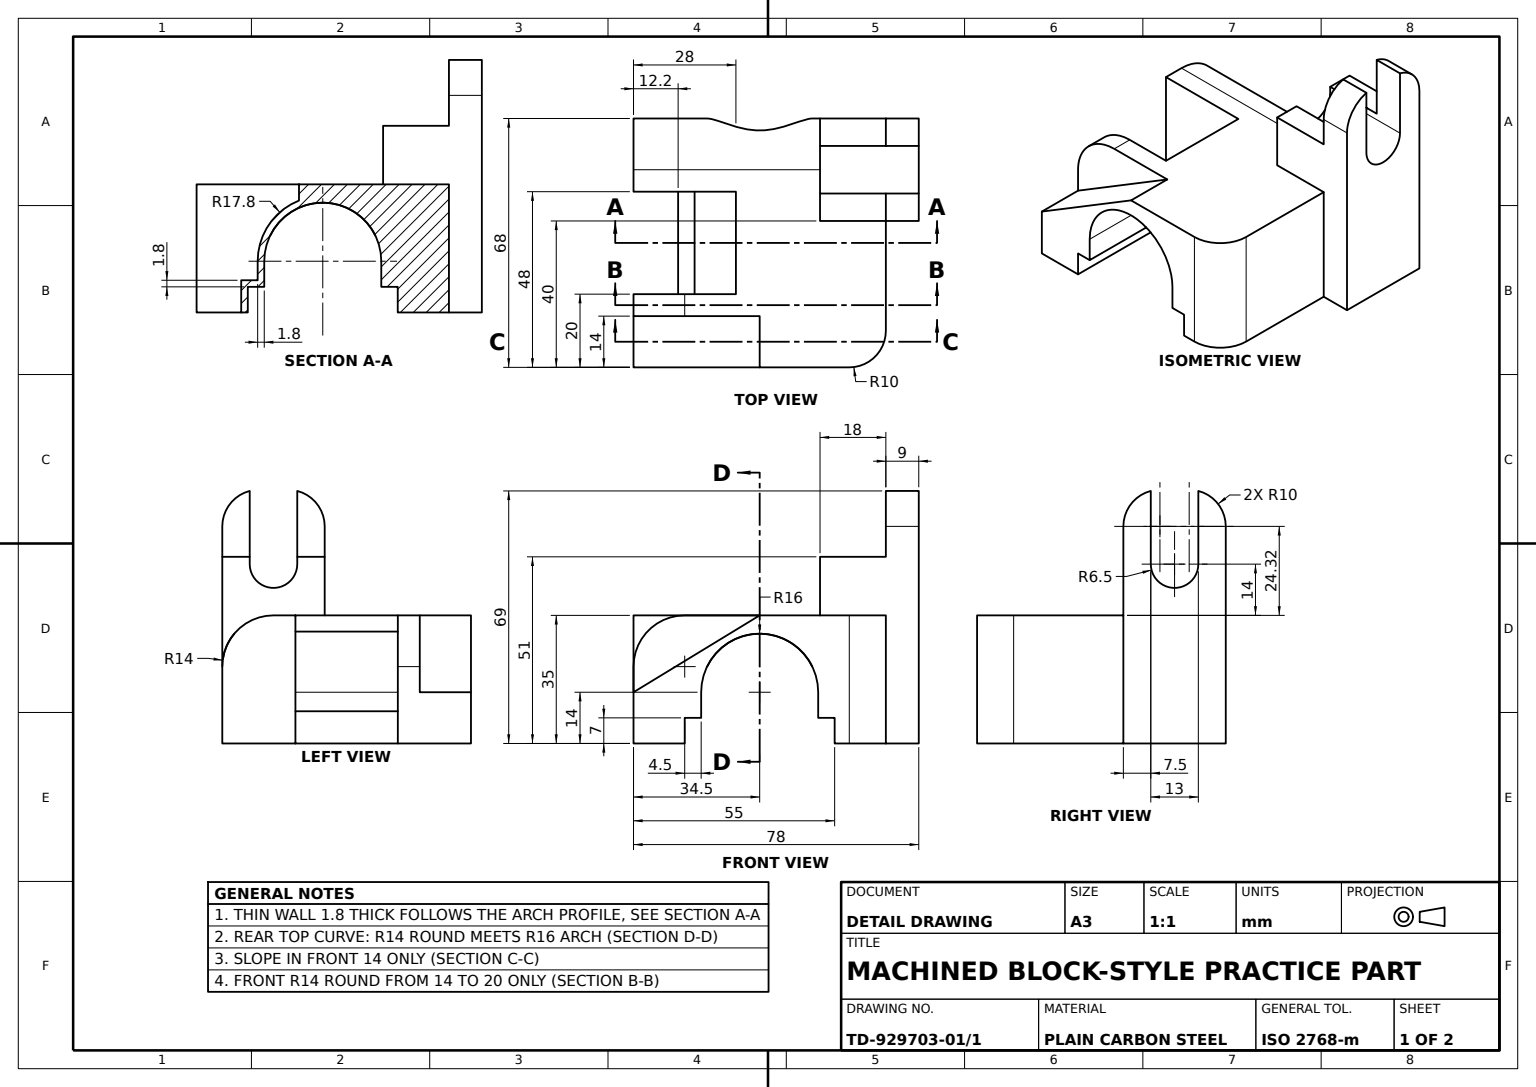
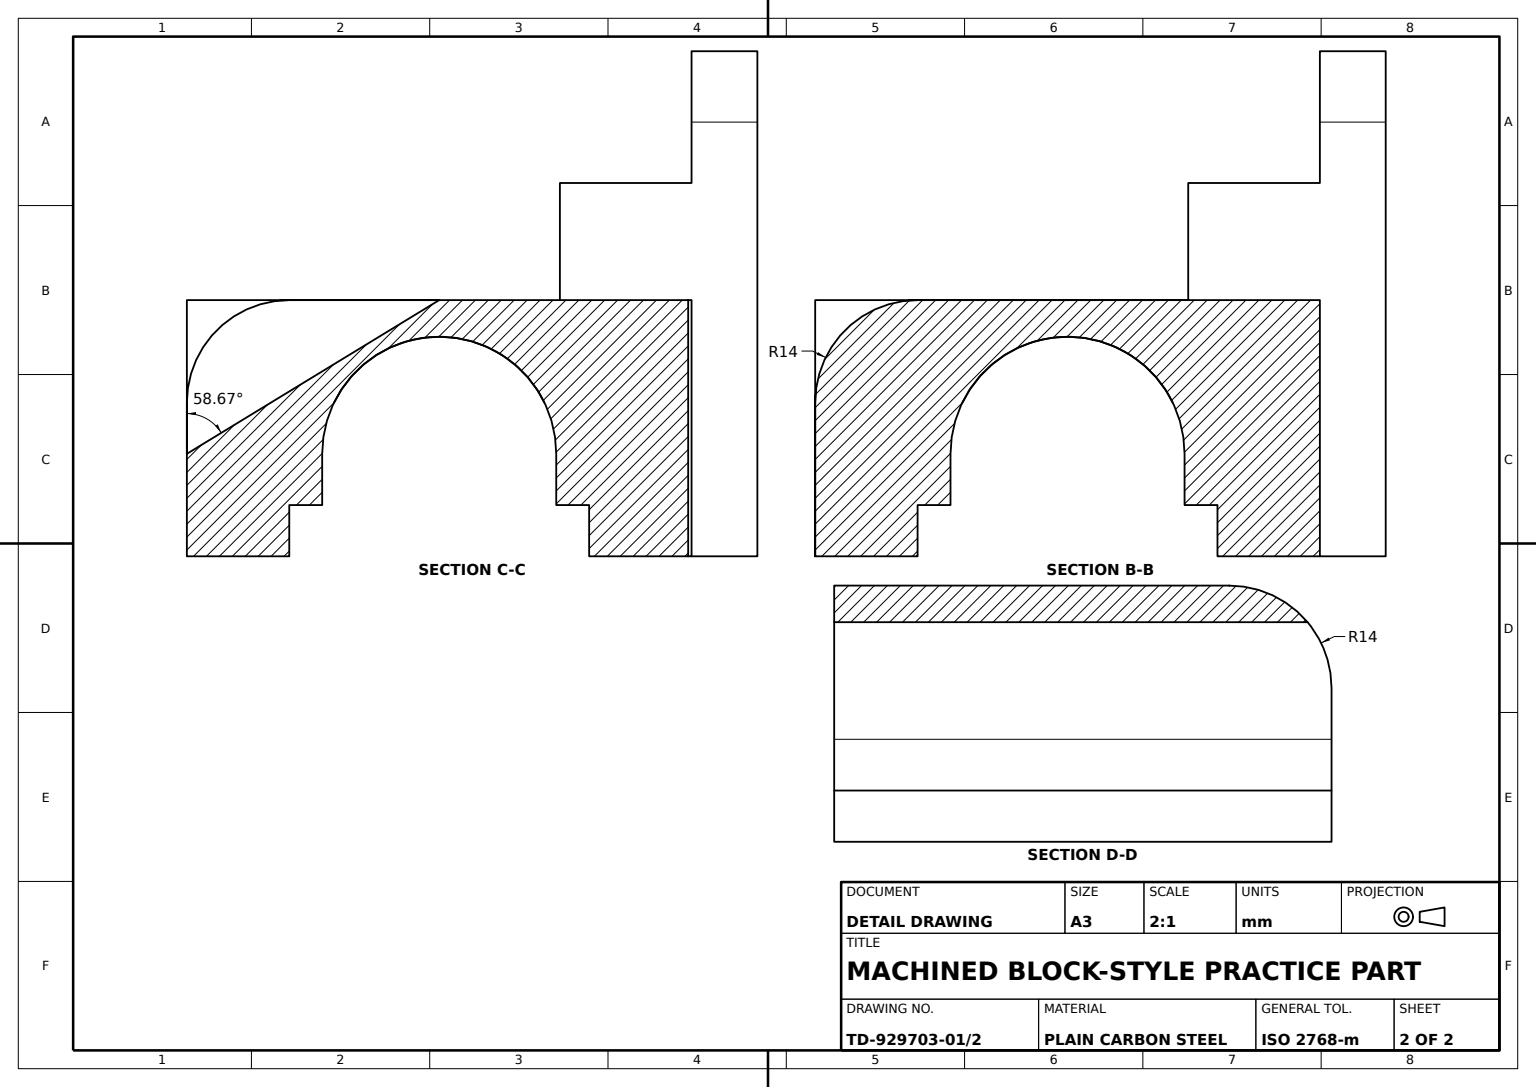
ISO-10303-21;
HEADER;
FILE_DESCRIPTION((''),'2;1');
FILE_NAME('','',(''),(''),'','','');
FILE_SCHEMA(('AUTOMOTIVE_DESIGN'));
ENDSEC;
DATA;
#1=APPLICATION_CONTEXT('');
#2=PRODUCT_CONTEXT('',#1,'mechanical');
#3=PRODUCT('','','',(#2));
#4=PRODUCT_DEFINITION_FORMATION('','',#3);
#5=PRODUCT_DEFINITION_CONTEXT('',#1,'design');
#6=PRODUCT_DEFINITION('','',#4,#5);
#7=PRODUCT_DEFINITION_SHAPE('','',#6);
#8=(LENGTH_UNIT()NAMED_UNIT(*)SI_UNIT(.MILLI.,.METRE.));
#9=(NAMED_UNIT(*)PLANE_ANGLE_UNIT()SI_UNIT($,.RADIAN.));
#10=(NAMED_UNIT(*)SI_UNIT($,.STERADIAN.)SOLID_ANGLE_UNIT());
#11=UNCERTAINTY_MEASURE_WITH_UNIT(LENGTH_MEASURE(1.E-05),#8,'distance_accuracy_value','');
#12=(GEOMETRIC_REPRESENTATION_CONTEXT(3)GLOBAL_UNCERTAINTY_ASSIGNED_CONTEXT((#11))GLOBAL_UNIT_ASSIGNED_CONTEXT((#8,#9,#10))REPRESENTATION_CONTEXT('',''));
#13=CARTESIAN_POINT('',(-28.,0.,22.3));
#14=VERTEX_POINT('',#13);
#15=CARTESIAN_POINT('',(-28.,0.,34.5));
#16=VERTEX_POINT('',#15);
#17=CARTESIAN_POINT('',(-28.,0.,-34.5));
#18=DIRECTION('',(0.,0.,1.));
#19=VECTOR('',#18,1000.);
#20=LINE('',#17,#19);
#21=EDGE_CURVE('',#14,#16,#20,.T.);
#22=ORIENTED_EDGE('',*,*,#21,.T.);
#23=CARTESIAN_POINT('',(-48.,0.,34.5));
#24=VERTEX_POINT('',#23);
#25=DIRECTION('',(1.,0.,0.));
#26=VECTOR('',#25,1000.);
#27=LINE('',#23,#26);
#28=EDGE_CURVE('',#24,#16,#27,.T.);
#29=ORIENTED_EDGE('',*,*,#28,.F.);
#30=CARTESIAN_POINT('',(-48.,0.,20.5));
#31=VERTEX_POINT('',#30);
#32=CARTESIAN_POINT('',(-48.,0.,22.3));
#33=DIRECTION('',(0.,0.,-1.));
#34=VECTOR('',#33,1000.);
#35=LINE('',#32,#34);
#36=EDGE_CURVE('',#24,#31,#35,.T.);
#37=ORIENTED_EDGE('',*,*,#36,.T.);
#38=CARTESIAN_POINT('',(20.,0.,20.5));
#39=VERTEX_POINT('',#38);
#40=DIRECTION('',(-1.,0.,0.));
#41=VECTOR('',#40,1000.);
#42=LINE('',#38,#41);
#43=EDGE_CURVE('',#39,#31,#42,.T.);
#44=ORIENTED_EDGE('',*,*,#43,.F.);
#45=CARTESIAN_POINT('',(20.,0.,34.5));
#46=VERTEX_POINT('',#45);
#47=LINE('',#38,#34);
#48=EDGE_CURVE('',#46,#39,#47,.T.);
#49=ORIENTED_EDGE('',*,*,#48,.F.);
#50=CARTESIAN_POINT('',(0.,0.,34.5));
#51=VERTEX_POINT('',#50);
#52=LINE('',#45,#41);
#53=EDGE_CURVE('',#46,#51,#52,.T.);
#54=ORIENTED_EDGE('',*,*,#53,.T.);
#55=CARTESIAN_POINT('',(0.,0.,22.3));
#56=VERTEX_POINT('',#55);
#57=CARTESIAN_POINT('',(0.,0.,20.5));
#58=LINE('',#57,#34);
#59=EDGE_CURVE('',#51,#56,#58,.T.);
#60=ORIENTED_EDGE('',*,*,#59,.T.);
#61=LINE('',#32,#26);
#62=EDGE_CURVE('',#14,#56,#61,.T.);
#63=ORIENTED_EDGE('',*,*,#62,.F.);
#64=EDGE_LOOP('',(#22,#29,#37,#44,#49,#54,#60,#63));
#65=FACE_OUTER_BOUND('',#64,.T.);
#66=DIRECTION('',(0.,1.,0.));
#67=AXIS2_PLACEMENT_3D('',#38,#66,#18);
#68=PLANE('',#67);
#69=ADVANCED_FACE('',(#65),#68,.F.);
#70=CARTESIAN_POINT('',(-34.,35.,-16.5));
#71=VERTEX_POINT('',#70);
#72=CARTESIAN_POINT('',(-34.,35.,34.5));
#73=VERTEX_POINT('',#72);
#74=CARTESIAN_POINT('',(-34.,35.,-34.5));
#75=LINE('',#74,#19);
#76=EDGE_CURVE('',#71,#73,#75,.T.);
#77=ORIENTED_EDGE('',*,*,#76,.F.);
#78=CARTESIAN_POINT('',(-48.,21.,-16.5));
#79=VERTEX_POINT('',#78);
#80=CARTESIAN_POINT('',(-34.,21.,-16.5));
#81=AXIS2_PLACEMENT_3D('',#80,#33,#40);
#82=CIRCLE('',#81,14.);
#83=EDGE_CURVE('',#79,#71,#82,.T.);
#84=ORIENTED_EDGE('',*,*,#83,.F.);
#85=CARTESIAN_POINT('',(-48.,21.,-14.387495));
#86=VERTEX_POINT('',#85);
#87=CARTESIAN_POINT('',(-48.,21.,-34.5));
#88=LINE('',#87,#19);
#89=EDGE_CURVE('',#79,#86,#88,.T.);
#90=ORIENTED_EDGE('',*,*,#89,.T.);
#91=CARTESIAN_POINT('',(-48.,21.,14.387495));
#92=VERTEX_POINT('',#91);
#93=CARTESIAN_POINT('',(-48.,21.691357,14.051126));
#94=CARTESIAN_POINT('',(-47.949279,22.345879,13.671469));
#95=CARTESIAN_POINT('',(-47.772933,23.588453,12.830602));
#96=CARTESIAN_POINT('',(-47.647073,24.176454,12.369366));
#97=CARTESIAN_POINT('',(-47.416507,25.010044,11.615476));
#98=CARTESIAN_POINT('',(-47.332968,25.2785,11.35485));
#99=CARTESIAN_POINT('',(-47.157195,25.79185,10.820788));
#100=CARTESIAN_POINT('',(-47.064704,26.037669,10.546527));
#101=CARTESIAN_POINT('',(-46.77748,26.744079,9.701921));
#102=CARTESIAN_POINT('',(-46.572941,27.173823,9.109937));
#103=CARTESIAN_POINT('',(-46.262441,27.758792,8.175009));
#104=CARTESIAN_POINT('',(-46.158355,27.94367,7.855474));
#105=CARTESIAN_POINT('',(-45.954634,28.288819,7.208609));
#106=CARTESIAN_POINT('',(-45.854643,28.449777,6.880233));
#107=CARTESIAN_POINT('',(-45.564597,28.898544,5.879459));
#108=CARTESIAN_POINT('',(-45.384364,29.152503,5.191539));
#109=CARTESIAN_POINT('',(-45.152422,29.464056,4.123175));
#110=CARTESIAN_POINT('',(-45.081534,29.556281,3.760943));
#111=CARTESIAN_POINT('',(-44.956058,29.716371,3.022951));
#112=CARTESIAN_POINT('',(-44.901811,29.78381,2.648455));
#113=CARTESIAN_POINT('',(-44.770586,29.945037,1.525661));
#114=CARTESIAN_POINT('',(-44.724263,29.999454,0.771499));
#115=CARTESIAN_POINT('',(-44.723354,30.000538,-0.748694));
#116=CARTESIAN_POINT('',(-44.770143,29.945562,-1.51979));
#117=CARTESIAN_POINT('',(-44.944464,29.731425,-3.015459));
#118=CARTESIAN_POINT('',(-45.071176,29.573011,-3.746822));
#119=CARTESIAN_POINT('',(-45.303955,29.260597,-4.82219));
#120=CARTESIAN_POINT('',(-45.389013,29.143396,-5.178379));
#121=CARTESIAN_POINT('',(-45.568252,28.886701,-5.875728));
#122=CARTESIAN_POINT('',(-45.662371,28.747324,-6.21698));
#123=CARTESIAN_POINT('',(-45.953336,28.296954,-7.220442));
#124=CARTESIAN_POINT('',(-46.158706,27.953947,-7.862507));
#125=CARTESIAN_POINT('',(-46.466645,27.374216,-8.789952));
#126=CARTESIAN_POINT('',(-46.569299,27.170045,-9.093118));
#127=CARTESIAN_POINT('',(-46.771892,26.738946,-9.687835));
#128=CARTESIAN_POINT('',(-46.872217,26.511031,-9.980509));
#129=CARTESIAN_POINT('',(-47.16131,25.800172,-10.830591));
#130=CARTESIAN_POINT('',(-47.338502,25.290303,-11.361077));
#131=CARTESIAN_POINT('',(-47.642102,24.196153,-12.352468));
#132=CARTESIAN_POINT('',(-47.768707,23.611927,-12.813378));
#133=CARTESIAN_POINT('',(-47.903214,22.673469,-13.450423));
#134=CARTESIAN_POINT('',(-47.938844,22.348842,-13.654447));
#135=CARTESIAN_POINT('',(-47.987191,21.685008,-14.038794));
#136=CARTESIAN_POINT('',(-48.,21.346074,-14.219118));
#137=B_SPLINE_CURVE_WITH_KNOTS('',3,(#91,#93,#94,#95,#96,#97,#98,#99,#100,#101,#102,#103,#104,#105,#106,#107,#108,#109,#110,#111,#112,#113,#114,#115,#116,#117,#118,#119,#120,#121,#122,#123,#124,#125,#126,#127,#128,#129,#130,#131,#132,#133,#134,#135,#136,#85),.UNSPECIFIED.,.F.,.F.,(4,2,2,2,2,2,2,2,2,2,2,2,2,2,2,2,2,2,2,2,2,2,4),(0.,0.002265979,0.004531958,0.005664947,0.006797937,0.009063916,0.010196905,0.011329895,0.013595874,0.014728863,0.015861853,0.018127832,0.02039381,0.022659789,0.023792779,0.024925768,0.027191747,0.028324737,0.029457726,0.031723705,0.033989684,0.035122674,0.036255663),.UNSPECIFIED.);
#138=EDGE_CURVE('',#92,#86,#137,.T.);
#139=ORIENTED_EDGE('',*,*,#138,.F.);
#140=CARTESIAN_POINT('',(-48.,21.,34.5));
#141=VERTEX_POINT('',#140);
#142=EDGE_CURVE('',#92,#141,#88,.T.);
#143=ORIENTED_EDGE('',*,*,#142,.T.);
#144=CARTESIAN_POINT('',(-34.,21.,34.5));
#145=AXIS2_PLACEMENT_3D('',#144,#18,#40);
#146=CIRCLE('',#145,14.);
#147=EDGE_CURVE('',#73,#141,#146,.T.);
#148=ORIENTED_EDGE('',*,*,#147,.F.);
#149=EDGE_LOOP('',(#77,#84,#90,#139,#143,#148));
#150=FACE_OUTER_BOUND('',#149,.T.);
#151=CARTESIAN_POINT('',(-34.,21.,-34.5));
#152=AXIS2_PLACEMENT_3D('',#151,#18,#25);
#153=CYLINDRICAL_SURFACE('',#152,14.);
#154=ADVANCED_FACE('',(#150),#153,.T.);
#155=CARTESIAN_POINT('',(20.,0.,-20.5));
#156=VERTEX_POINT('',#155);
#157=CARTESIAN_POINT('',(-48.,0.,-20.5));
#158=VERTEX_POINT('',#157);
#159=LINE('',#155,#41);
#160=EDGE_CURVE('',#156,#158,#159,.T.);
#161=ORIENTED_EDGE('',*,*,#160,.F.);
#162=CARTESIAN_POINT('',(20.,7.,-20.5));
#163=VERTEX_POINT('',#162);
#164=DIRECTION('',(0.,-1.,0.));
#165=VECTOR('',#164,1000.);
#166=LINE('',#155,#165);
#167=EDGE_CURVE('',#163,#156,#166,.T.);
#168=ORIENTED_EDGE('',*,*,#167,.F.);
#169=CARTESIAN_POINT('',(-48.,7.,-20.5));
#170=VERTEX_POINT('',#169);
#171=LINE('',#162,#41);
#172=EDGE_CURVE('',#163,#170,#171,.T.);
#173=ORIENTED_EDGE('',*,*,#172,.T.);
#174=CARTESIAN_POINT('',(-48.,14.,-20.5));
#175=LINE('',#174,#165);
#176=EDGE_CURVE('',#170,#158,#175,.T.);
#177=ORIENTED_EDGE('',*,*,#176,.T.);
#178=EDGE_LOOP('',(#161,#168,#173,#177));
#179=FACE_OUTER_BOUND('',#178,.T.);
#180=AXIS2_PLACEMENT_3D('',#155,#33,#40);
#181=PLANE('',#180);
#182=ADVANCED_FACE('',(#179),#181,.F.);
#183=CARTESIAN_POINT('',(20.,35.,-24.5));
#184=VERTEX_POINT('',#183);
#185=CARTESIAN_POINT('',(20.,35.,0.));
#186=VERTEX_POINT('',#185);
#187=CARTESIAN_POINT('',(20.,35.,20.5));
#188=LINE('',#187,#19);
#189=EDGE_CURVE('',#184,#186,#188,.T.);
#190=ORIENTED_EDGE('',*,*,#189,.T.);
#191=CARTESIAN_POINT('',(20.,14.,34.5));
#192=VERTEX_POINT('',#191);
#193=DIRECTION('',(0.,0.519946947,-0.854198556));
#194=VECTOR('',#193,1000.);
#195=LINE('',#191,#194);
#196=EDGE_CURVE('',#192,#186,#195,.T.);
#197=ORIENTED_EDGE('',*,*,#196,.F.);
#198=LINE('',#45,#165);
#199=EDGE_CURVE('',#192,#46,#198,.T.);
#200=ORIENTED_EDGE('',*,*,#199,.T.);
#201=ORIENTED_EDGE('',*,*,#48,.T.);
#202=CARTESIAN_POINT('',(20.,7.,20.5));
#203=VERTEX_POINT('',#202);
#204=VECTOR('',#66,1000.);
#205=LINE('',#202,#204);
#206=EDGE_CURVE('',#39,#203,#205,.T.);
#207=ORIENTED_EDGE('',*,*,#206,.T.);
#208=CARTESIAN_POINT('',(20.,7.,16.));
#209=VERTEX_POINT('',#208);
#210=LINE('',#208,#34);
#211=EDGE_CURVE('',#203,#209,#210,.T.);
#212=ORIENTED_EDGE('',*,*,#211,.T.);
#213=CARTESIAN_POINT('',(20.,14.,16.));
#214=VERTEX_POINT('',#213);
#215=LINE('',#213,#204);
#216=EDGE_CURVE('',#209,#214,#215,.T.);
#217=ORIENTED_EDGE('',*,*,#216,.T.);
#218=CARTESIAN_POINT('',(20.,14.,-16.));
#219=VERTEX_POINT('',#218);
#220=CARTESIAN_POINT('',(20.,14.,0.));
#221=AXIS2_PLACEMENT_3D('',#220,#40,#33);
#222=CIRCLE('',#221,16.);
#223=EDGE_CURVE('',#214,#219,#222,.T.);
#224=ORIENTED_EDGE('',*,*,#223,.T.);
#225=CARTESIAN_POINT('',(20.,7.,-16.));
#226=VERTEX_POINT('',#225);
#227=LINE('',#218,#165);
#228=EDGE_CURVE('',#219,#226,#227,.T.);
#229=ORIENTED_EDGE('',*,*,#228,.T.);
#230=LINE('',#225,#34);
#231=EDGE_CURVE('',#226,#163,#230,.T.);
#232=ORIENTED_EDGE('',*,*,#231,.T.);
#233=ORIENTED_EDGE('',*,*,#167,.T.);
#234=CARTESIAN_POINT('',(20.,0.,-24.5));
#235=VERTEX_POINT('',#234);
#236=CARTESIAN_POINT('',(20.,0.,-34.5));
#237=LINE('',#236,#34);
#238=EDGE_CURVE('',#156,#235,#237,.T.);
#239=ORIENTED_EDGE('',*,*,#238,.T.);
#240=LINE('',#183,#204);
#241=EDGE_CURVE('',#235,#184,#240,.T.);
#242=ORIENTED_EDGE('',*,*,#241,.T.);
#243=EDGE_LOOP('',(#190,#197,#200,#201,#207,#212,#217,#224,#229,#232,#233,#239,#242));
#244=FACE_OUTER_BOUND('',#243,.T.);
#245=AXIS2_PLACEMENT_3D('',#220,#25,#33);
#246=PLANE('',#245);
#247=ADVANCED_FACE('',(#244),#246,.T.);
#248=CARTESIAN_POINT('',(10.,0.,-34.5));
#249=VERTEX_POINT('',#248);
#250=CARTESIAN_POINT('',(-20.,0.,-34.5));
#251=VERTEX_POINT('',#250);
#252=LINE('',#236,#41);
#253=EDGE_CURVE('',#249,#251,#252,.T.);
#254=ORIENTED_EDGE('',*,*,#253,.T.);
#255=CARTESIAN_POINT('',(-20.,35.,-34.5));
#256=VERTEX_POINT('',#255);
#257=CARTESIAN_POINT('',(-20.,21.,-34.5));
#258=LINE('',#257,#165);
#259=EDGE_CURVE('',#256,#251,#258,.T.);
#260=ORIENTED_EDGE('',*,*,#259,.F.);
#261=CARTESIAN_POINT('',(10.,35.,-34.5));
#262=VERTEX_POINT('',#261);
#263=CARTESIAN_POINT('',(20.,35.,-34.5));
#264=LINE('',#263,#41);
#265=EDGE_CURVE('',#262,#256,#264,.T.);
#266=ORIENTED_EDGE('',*,*,#265,.F.);
#267=LINE('',#248,#165);
#268=EDGE_CURVE('',#262,#249,#267,.T.);
#269=ORIENTED_EDGE('',*,*,#268,.T.);
#270=EDGE_LOOP('',(#254,#260,#266,#269));
#271=FACE_OUTER_BOUND('',#270,.T.);
#272=AXIS2_PLACEMENT_3D('',#263,#18,#25);
#273=PLANE('',#272);
#274=ADVANCED_FACE('',(#271),#273,.F.);
#275=CARTESIAN_POINT('',(6.,35.,0.));
#276=VERTEX_POINT('',#275);
#277=LINE('',#275,#26);
#278=EDGE_CURVE('',#276,#186,#277,.T.);
#279=ORIENTED_EDGE('',*,*,#278,.T.);
#280=ORIENTED_EDGE('',*,*,#189,.F.);
#281=CARTESIAN_POINT('',(10.,35.,-24.5));
#282=AXIS2_PLACEMENT_3D('',#281,#66,#33);
#283=CIRCLE('',#282,10.);
#284=EDGE_CURVE('',#184,#262,#283,.T.);
#285=ORIENTED_EDGE('',*,*,#284,.T.);
#286=ORIENTED_EDGE('',*,*,#265,.T.);
#287=CARTESIAN_POINT('',(-20.,35.,-16.5));
#288=VERTEX_POINT('',#287);
#289=LINE('',#287,#34);
#290=EDGE_CURVE('',#288,#256,#289,.T.);
#291=ORIENTED_EDGE('',*,*,#290,.F.);
#292=LINE('',#70,#26);
#293=EDGE_CURVE('',#71,#288,#292,.T.);
#294=ORIENTED_EDGE('',*,*,#293,.F.);
#295=ORIENTED_EDGE('',*,*,#76,.T.);
#296=CARTESIAN_POINT('',(-28.,35.,34.5));
#297=VERTEX_POINT('',#296);
#298=LINE('',#296,#41);
#299=EDGE_CURVE('',#297,#73,#298,.T.);
#300=ORIENTED_EDGE('',*,*,#299,.F.);
#301=CARTESIAN_POINT('',(-28.,35.,6.5));
#302=VERTEX_POINT('',#301);
#303=CARTESIAN_POINT('',(-28.,35.,-34.5));
#304=LINE('',#303,#19);
#305=EDGE_CURVE('',#302,#297,#304,.T.);
#306=ORIENTED_EDGE('',*,*,#305,.F.);
#307=CARTESIAN_POINT('',(0.,35.,6.5));
#308=VERTEX_POINT('',#307);
#309=LINE('',#307,#26);
#310=EDGE_CURVE('',#302,#308,#309,.T.);
#311=ORIENTED_EDGE('',*,*,#310,.T.);
#312=CARTESIAN_POINT('',(0.,35.,20.5));
#313=VERTEX_POINT('',#312);
#314=LINE('',#312,#19);
#315=EDGE_CURVE('',#308,#313,#314,.T.);
#316=ORIENTED_EDGE('',*,*,#315,.T.);
#317=CARTESIAN_POINT('',(6.,35.,20.5));
#318=VERTEX_POINT('',#317);
#319=LINE('',#187,#41);
#320=EDGE_CURVE('',#318,#313,#319,.T.);
#321=ORIENTED_EDGE('',*,*,#320,.F.);
#322=LINE('',#317,#19);
#323=EDGE_CURVE('',#276,#318,#322,.T.);
#324=ORIENTED_EDGE('',*,*,#323,.F.);
#325=EDGE_LOOP('',(#279,#280,#285,#286,#291,#294,#295,#300,#306,#311,#316,#321,#324));
#326=FACE_OUTER_BOUND('',#325,.T.);
#327=AXIS2_PLACEMENT_3D('',#187,#164,#33);
#328=PLANE('',#327);
#329=ADVANCED_FACE('',(#326),#328,.F.);
#330=CARTESIAN_POINT('',(-27.5,69.,-34.5));
#331=VERTEX_POINT('',#330);
#332=CARTESIAN_POINT('',(-20.,59.317542,-34.5));
#333=VERTEX_POINT('',#332);
#334=CARTESIAN_POINT('',(-30.,59.317542,-34.5));
#335=AXIS2_PLACEMENT_3D('',#334,#33,#40);
#336=CIRCLE('',#335,10.);
#337=EDGE_CURVE('',#331,#333,#336,.T.);
#338=ORIENTED_EDGE('',*,*,#337,.F.);
#339=CARTESIAN_POINT('',(-27.5,51.,-34.5));
#340=VERTEX_POINT('',#339);
#341=CARTESIAN_POINT('',(-27.5,49.,-34.5));
#342=LINE('',#341,#204);
#343=EDGE_CURVE('',#340,#331,#342,.T.);
#344=ORIENTED_EDGE('',*,*,#343,.F.);
#345=CARTESIAN_POINT('',(-20.,51.,-34.5));
#346=VERTEX_POINT('',#345);
#347=LINE('',#339,#41);
#348=EDGE_CURVE('',#346,#340,#347,.T.);
#349=ORIENTED_EDGE('',*,*,#348,.F.);
#350=EDGE_CURVE('',#333,#346,#258,.T.);
#351=ORIENTED_EDGE('',*,*,#350,.F.);
#352=EDGE_LOOP('',(#338,#344,#349,#351));
#353=FACE_OUTER_BOUND('',#352,.T.);
#354=CARTESIAN_POINT('',(-38.,59.317542,-34.5));
#355=AXIS2_PLACEMENT_3D('',#354,#18,#25);
#356=PLANE('',#355);
#357=ADVANCED_FACE('',(#353),#356,.T.);
#358=CARTESIAN_POINT('',(-48.,7.,16.));
#359=VERTEX_POINT('',#358);
#360=LINE('',#208,#41);
#361=EDGE_CURVE('',#209,#359,#360,.T.);
#362=ORIENTED_EDGE('',*,*,#361,.F.);
#363=ORIENTED_EDGE('',*,*,#211,.F.);
#364=CARTESIAN_POINT('',(-48.,7.,20.5));
#365=VERTEX_POINT('',#364);
#366=LINE('',#202,#41);
#367=EDGE_CURVE('',#203,#365,#366,.T.);
#368=ORIENTED_EDGE('',*,*,#367,.T.);
#369=CARTESIAN_POINT('',(-48.,7.,0.));
#370=LINE('',#369,#34);
#371=EDGE_CURVE('',#365,#359,#370,.T.);
#372=ORIENTED_EDGE('',*,*,#371,.T.);
#373=EDGE_LOOP('',(#362,#363,#368,#372));
#374=FACE_OUTER_BOUND('',#373,.T.);
#375=AXIS2_PLACEMENT_3D('',#208,#66,#18);
#376=PLANE('',#375);
#377=ADVANCED_FACE('',(#374),#376,.F.);
#378=CARTESIAN_POINT('',(-48.,0.,-43.5));
#379=VERTEX_POINT('',#378);
#380=EDGE_CURVE('',#158,#379,#35,.T.);
#381=ORIENTED_EDGE('',*,*,#380,.F.);
#382=ORIENTED_EDGE('',*,*,#176,.F.);
#383=CARTESIAN_POINT('',(-48.,7.,-16.));
#384=VERTEX_POINT('',#383);
#385=EDGE_CURVE('',#384,#170,#370,.T.);
#386=ORIENTED_EDGE('',*,*,#385,.F.);
#387=CARTESIAN_POINT('',(-48.,14.,-16.));
#388=VERTEX_POINT('',#387);
#389=LINE('',#387,#165);
#390=EDGE_CURVE('',#388,#384,#389,.T.);
#391=ORIENTED_EDGE('',*,*,#390,.F.);
#392=CARTESIAN_POINT('',(-48.,14.,0.));
#393=AXIS2_PLACEMENT_3D('',#392,#40,#18);
#394=CIRCLE('',#393,16.);
#395=EDGE_CURVE('',#86,#388,#394,.T.);
#396=ORIENTED_EDGE('',*,*,#395,.F.);
#397=ORIENTED_EDGE('',*,*,#89,.F.);
#398=CARTESIAN_POINT('',(-48.,51.,-16.5));
#399=VERTEX_POINT('',#398);
#400=LINE('',#398,#165);
#401=EDGE_CURVE('',#399,#79,#400,.T.);
#402=ORIENTED_EDGE('',*,*,#401,.F.);
#403=CARTESIAN_POINT('',(-48.,51.,-34.5));
#404=VERTEX_POINT('',#403);
#405=LINE('',#398,#34);
#406=EDGE_CURVE('',#399,#404,#405,.T.);
#407=ORIENTED_EDGE('',*,*,#406,.T.);
#408=CARTESIAN_POINT('',(-48.,59.317542,-34.5));
#409=VERTEX_POINT('',#408);
#410=LINE('',#408,#204);
#411=EDGE_CURVE('',#404,#409,#410,.T.);
#412=ORIENTED_EDGE('',*,*,#411,.T.);
#413=CARTESIAN_POINT('',(-48.,59.317542,-43.5));
#414=VERTEX_POINT('',#413);
#415=LINE('',#413,#19);
#416=EDGE_CURVE('',#414,#409,#415,.T.);
#417=ORIENTED_EDGE('',*,*,#416,.F.);
#418=LINE('',#378,#204);
#419=EDGE_CURVE('',#379,#414,#418,.T.);
#420=ORIENTED_EDGE('',*,*,#419,.F.);
#421=EDGE_LOOP('',(#381,#382,#386,#391,#396,#397,#402,#407,#412,#417,#420));
#422=FACE_OUTER_BOUND('',#421,.T.);
#423=PLANE('',#393);
#424=ADVANCED_FACE('',(#422),#423,.T.);
#425=LINE('',#23,#165);
#426=EDGE_CURVE('',#141,#24,#425,.T.);
#427=ORIENTED_EDGE('',*,*,#426,.F.);
#428=ORIENTED_EDGE('',*,*,#142,.F.);
#429=CARTESIAN_POINT('',(-48.,14.,16.));
#430=VERTEX_POINT('',#429);
#431=EDGE_CURVE('',#430,#92,#394,.T.);
#432=ORIENTED_EDGE('',*,*,#431,.F.);
#433=LINE('',#429,#204);
#434=EDGE_CURVE('',#359,#430,#433,.T.);
#435=ORIENTED_EDGE('',*,*,#434,.F.);
#436=ORIENTED_EDGE('',*,*,#371,.F.);
#437=CARTESIAN_POINT('',(-48.,14.,20.5));
#438=LINE('',#437,#204);
#439=EDGE_CURVE('',#31,#365,#438,.T.);
#440=ORIENTED_EDGE('',*,*,#439,.F.);
#441=ORIENTED_EDGE('',*,*,#36,.F.);
#442=EDGE_LOOP('',(#427,#428,#432,#435,#436,#440,#441));
#443=FACE_OUTER_BOUND('',#442,.T.);
#444=ADVANCED_FACE('',(#443),#423,.T.);
#445=ORIENTED_EDGE('',*,*,#62,.T.);
#446=CARTESIAN_POINT('',(0.,8.8,22.3));
#447=VERTEX_POINT('',#446);
#448=CARTESIAN_POINT('',(0.,14.,22.3));
#449=LINE('',#448,#165);
#450=EDGE_CURVE('',#447,#56,#449,.T.);
#451=ORIENTED_EDGE('',*,*,#450,.F.);
#452=CARTESIAN_POINT('',(-28.,8.8,22.3));
#453=VERTEX_POINT('',#452);
#454=CARTESIAN_POINT('',(-48.,8.8,22.3));
#455=LINE('',#454,#26);
#456=EDGE_CURVE('',#453,#447,#455,.T.);
#457=ORIENTED_EDGE('',*,*,#456,.F.);
#458=LINE('',#452,#204);
#459=EDGE_CURVE('',#14,#453,#458,.T.);
#460=ORIENTED_EDGE('',*,*,#459,.F.);
#461=EDGE_LOOP('',(#445,#451,#457,#460));
#462=FACE_OUTER_BOUND('',#461,.T.);
#463=AXIS2_PLACEMENT_3D('',#454,#18,#25);
#464=PLANE('',#463);
#465=ADVANCED_FACE('',(#462),#464,.T.);
#466=CARTESIAN_POINT('',(6.,14.,34.5));
#467=VERTEX_POINT('',#466);
#468=LINE('',#466,#26);
#469=EDGE_CURVE('',#467,#192,#468,.T.);
#470=ORIENTED_EDGE('',*,*,#469,.T.);
#471=ORIENTED_EDGE('',*,*,#196,.T.);
#472=ORIENTED_EDGE('',*,*,#278,.F.);
#473=LINE('',#466,#194);
#474=EDGE_CURVE('',#467,#276,#473,.T.);
#475=ORIENTED_EDGE('',*,*,#474,.F.);
#476=EDGE_LOOP('',(#470,#471,#472,#475));
#477=FACE_OUTER_BOUND('',#476,.T.);
#478=DIRECTION('',(0.,-0.854198556,-0.519946947));
#479=AXIS2_PLACEMENT_3D('',#466,#478,#193);
#480=PLANE('',#479);
#481=ADVANCED_FACE('',(#477),#480,.F.);
#482=LINE('',#218,#41);
#483=EDGE_CURVE('',#219,#388,#482,.T.);
#484=ORIENTED_EDGE('',*,*,#483,.T.);
#485=ORIENTED_EDGE('',*,*,#390,.T.);
#486=LINE('',#225,#41);
#487=EDGE_CURVE('',#226,#384,#486,.T.);
#488=ORIENTED_EDGE('',*,*,#487,.F.);
#489=ORIENTED_EDGE('',*,*,#228,.F.);
#490=EDGE_LOOP('',(#484,#485,#488,#489));
#491=FACE_OUTER_BOUND('',#490,.T.);
#492=AXIS2_PLACEMENT_3D('',#218,#33,#66);
#493=PLANE('',#492);
#494=ADVANCED_FACE('',(#491),#493,.F.);
#495=CARTESIAN_POINT('',(0.,21.,34.5));
#496=VERTEX_POINT('',#495);
#497=LINE('',#50,#165);
#498=EDGE_CURVE('',#496,#51,#497,.T.);
#499=ORIENTED_EDGE('',*,*,#498,.T.);
#500=ORIENTED_EDGE('',*,*,#53,.F.);
#501=ORIENTED_EDGE('',*,*,#199,.F.);
#502=ORIENTED_EDGE('',*,*,#469,.F.);
#503=CARTESIAN_POINT('',(6.,21.,34.5));
#504=VERTEX_POINT('',#503);
#505=LINE('',#503,#165);
#506=EDGE_CURVE('',#504,#467,#505,.T.);
#507=ORIENTED_EDGE('',*,*,#506,.F.);
#508=CARTESIAN_POINT('',(20.,21.,34.5));
#509=LINE('',#508,#41);
#510=EDGE_CURVE('',#504,#496,#509,.T.);
#511=ORIENTED_EDGE('',*,*,#510,.T.);
#512=EDGE_LOOP('',(#499,#500,#501,#502,#507,#511));
#513=FACE_OUTER_BOUND('',#512,.T.);
#514=AXIS2_PLACEMENT_3D('',#45,#33,#40);
#515=PLANE('',#514);
#516=ADVANCED_FACE('',(#513),#515,.F.);
#517=CARTESIAN_POINT('',(-28.,8.8,17.8));
#518=VERTEX_POINT('',#517);
#519=CARTESIAN_POINT('',(0.,8.8,17.8));
#520=VERTEX_POINT('',#519);
#521=CARTESIAN_POINT('',(-48.,8.8,17.8));
#522=LINE('',#521,#26);
#523=EDGE_CURVE('',#518,#520,#522,.T.);
#524=ORIENTED_EDGE('',*,*,#523,.T.);
#525=CARTESIAN_POINT('',(0.,14.,17.8));
#526=VERTEX_POINT('',#525);
#527=LINE('',#525,#165);
#528=EDGE_CURVE('',#526,#520,#527,.T.);
#529=ORIENTED_EDGE('',*,*,#528,.F.);
#530=CARTESIAN_POINT('',(-28.,14.,17.8));
#531=VERTEX_POINT('',#530);
#532=CARTESIAN_POINT('',(-48.,14.,17.8));
#533=LINE('',#532,#26);
#534=EDGE_CURVE('',#531,#526,#533,.T.);
#535=ORIENTED_EDGE('',*,*,#534,.F.);
#536=LINE('',#530,#204);
#537=EDGE_CURVE('',#518,#531,#536,.T.);
#538=ORIENTED_EDGE('',*,*,#537,.F.);
#539=EDGE_LOOP('',(#524,#529,#535,#538));
#540=FACE_OUTER_BOUND('',#539,.T.);
#541=AXIS2_PLACEMENT_3D('',#532,#18,#25);
#542=PLANE('',#541);
#543=ADVANCED_FACE('',(#540),#542,.T.);
#544=ORIENTED_EDGE('',*,*,#147,.T.);
#545=ORIENTED_EDGE('',*,*,#426,.T.);
#546=ORIENTED_EDGE('',*,*,#28,.T.);
#547=LINE('',#15,#204);
#548=EDGE_CURVE('',#16,#297,#547,.T.);
#549=ORIENTED_EDGE('',*,*,#548,.T.);
#550=ORIENTED_EDGE('',*,*,#299,.T.);
#551=EDGE_LOOP('',(#544,#545,#546,#549,#550));
#552=FACE_OUTER_BOUND('',#551,.T.);
#553=AXIS2_PLACEMENT_3D('',#144,#33,#40);
#554=PLANE('',#553);
#555=ADVANCED_FACE('',(#552),#554,.F.);
#556=ORIENTED_EDGE('',*,*,#439,.T.);
#557=ORIENTED_EDGE('',*,*,#367,.F.);
#558=ORIENTED_EDGE('',*,*,#206,.F.);
#559=ORIENTED_EDGE('',*,*,#43,.T.);
#560=EDGE_LOOP('',(#556,#557,#558,#559));
#561=FACE_OUTER_BOUND('',#560,.T.);
#562=AXIS2_PLACEMENT_3D('',#202,#18,#25);
#563=PLANE('',#562);
#564=ADVANCED_FACE('',(#561),#563,.F.);
#565=ORIENTED_EDGE('',*,*,#416,.T.);
#566=CARTESIAN_POINT('',(-40.5,69.,-34.5));
#567=VERTEX_POINT('',#566);
#568=AXIS2_PLACEMENT_3D('',#354,#33,#25);
#569=CIRCLE('',#568,10.);
#570=EDGE_CURVE('',#409,#567,#569,.T.);
#571=ORIENTED_EDGE('',*,*,#570,.T.);
#572=CARTESIAN_POINT('',(-40.5,69.,-43.5));
#573=VERTEX_POINT('',#572);
#574=LINE('',#572,#19);
#575=EDGE_CURVE('',#573,#567,#574,.T.);
#576=ORIENTED_EDGE('',*,*,#575,.F.);
#577=CARTESIAN_POINT('',(-38.,59.317542,-43.5));
#578=AXIS2_PLACEMENT_3D('',#577,#33,#25);
#579=CIRCLE('',#578,10.);
#580=EDGE_CURVE('',#414,#573,#579,.T.);
#581=ORIENTED_EDGE('',*,*,#580,.F.);
#582=EDGE_LOOP('',(#565,#571,#576,#581));
#583=FACE_OUTER_BOUND('',#582,.T.);
#584=AXIS2_PLACEMENT_3D('',#577,#18,#25);
#585=CYLINDRICAL_SURFACE('',#584,10.);
#586=ADVANCED_FACE('',(#583),#585,.T.);
#587=CARTESIAN_POINT('',(-40.5,49.,-16.5));
#588=VERTEX_POINT('',#587);
#589=CARTESIAN_POINT('',(-40.5,51.,-16.5));
#590=VERTEX_POINT('',#589);
#591=LINE('',#587,#204);
#592=EDGE_CURVE('',#588,#590,#591,.T.);
#593=ORIENTED_EDGE('',*,*,#592,.T.);
#594=LINE('',#589,#41);
#595=EDGE_CURVE('',#590,#399,#594,.T.);
#596=ORIENTED_EDGE('',*,*,#595,.T.);
#597=ORIENTED_EDGE('',*,*,#401,.T.);
#598=ORIENTED_EDGE('',*,*,#83,.T.);
#599=ORIENTED_EDGE('',*,*,#293,.T.);
#600=CARTESIAN_POINT('',(-20.,51.,-16.5));
#601=VERTEX_POINT('',#600);
#602=LINE('',#287,#204);
#603=EDGE_CURVE('',#288,#601,#602,.T.);
#604=ORIENTED_EDGE('',*,*,#603,.T.);
#605=CARTESIAN_POINT('',(-27.5,51.,-16.5));
#606=VERTEX_POINT('',#605);
#607=LINE('',#605,#41);
#608=EDGE_CURVE('',#601,#606,#607,.T.);
#609=ORIENTED_EDGE('',*,*,#608,.T.);
#610=CARTESIAN_POINT('',(-27.5,49.,-16.5));
#611=VERTEX_POINT('',#610);
#612=LINE('',#610,#165);
#613=EDGE_CURVE('',#606,#611,#612,.T.);
#614=ORIENTED_EDGE('',*,*,#613,.T.);
#615=CARTESIAN_POINT('',(-34.,49.,-16.5));
#616=AXIS2_PLACEMENT_3D('',#615,#33,#25);
#617=CIRCLE('',#616,6.5);
#618=EDGE_CURVE('',#611,#588,#617,.T.);
#619=ORIENTED_EDGE('',*,*,#618,.T.);
#620=EDGE_LOOP('',(#593,#596,#597,#598,#599,#604,#609,#614,#619));
#621=FACE_OUTER_BOUND('',#620,.T.);
#622=AXIS2_PLACEMENT_3D('',#615,#18,#25);
#623=PLANE('',#622);
#624=ADVANCED_FACE('',(#621),#623,.T.);
#625=CARTESIAN_POINT('',(-40.5,49.,-43.5));
#626=VERTEX_POINT('',#625);
#627=LINE('',#625,#19);
#628=EDGE_CURVE('',#626,#588,#627,.T.);
#629=ORIENTED_EDGE('',*,*,#628,.T.);
#630=ORIENTED_EDGE('',*,*,#618,.F.);
#631=CARTESIAN_POINT('',(-27.5,49.,-43.5));
#632=VERTEX_POINT('',#631);
#633=LINE('',#631,#19);
#634=EDGE_CURVE('',#632,#611,#633,.T.);
#635=ORIENTED_EDGE('',*,*,#634,.F.);
#636=CARTESIAN_POINT('',(-34.,49.,-43.5));
#637=AXIS2_PLACEMENT_3D('',#636,#18,#40);
#638=CIRCLE('',#637,6.5);
#639=EDGE_CURVE('',#626,#632,#638,.T.);
#640=ORIENTED_EDGE('',*,*,#639,.F.);
#641=EDGE_LOOP('',(#629,#630,#635,#640));
#642=FACE_OUTER_BOUND('',#641,.T.);
#643=AXIS2_PLACEMENT_3D('',#636,#18,#25);
#644=CYLINDRICAL_SURFACE('',#643,6.5);
#645=ADVANCED_FACE('',(#642),#644,.F.);
#646=ORIENTED_EDGE('',*,*,#608,.F.);
#647=LINE('',#600,#34);
#648=EDGE_CURVE('',#601,#346,#647,.T.);
#649=ORIENTED_EDGE('',*,*,#648,.T.);
#650=ORIENTED_EDGE('',*,*,#348,.T.);
#651=LINE('',#605,#34);
#652=EDGE_CURVE('',#606,#340,#651,.T.);
#653=ORIENTED_EDGE('',*,*,#652,.F.);
#654=EDGE_LOOP('',(#646,#649,#650,#653));
#655=FACE_OUTER_BOUND('',#654,.T.);
#656=AXIS2_PLACEMENT_3D('',#605,#164,#33);
#657=PLANE('',#656);
#658=ADVANCED_FACE('',(#655),#657,.F.);
#659=ORIENTED_EDGE('',*,*,#172,.F.);
#660=ORIENTED_EDGE('',*,*,#231,.F.);
#661=ORIENTED_EDGE('',*,*,#487,.T.);
#662=ORIENTED_EDGE('',*,*,#385,.T.);
#663=EDGE_LOOP('',(#659,#660,#661,#662));
#664=FACE_OUTER_BOUND('',#663,.T.);
#665=AXIS2_PLACEMENT_3D('',#225,#66,#18);
#666=PLANE('',#665);
#667=ADVANCED_FACE('',(#664),#666,.F.);
#668=CARTESIAN_POINT('',(6.,21.,20.5));
#669=AXIS2_PLACEMENT_3D('',#668,#25,#18);
#670=CIRCLE('',#669,14.);
#671=EDGE_CURVE('',#318,#504,#670,.T.);
#672=ORIENTED_EDGE('',*,*,#671,.T.);
#673=ORIENTED_EDGE('',*,*,#506,.T.);
#674=ORIENTED_EDGE('',*,*,#474,.T.);
#675=ORIENTED_EDGE('',*,*,#323,.T.);
#676=EDGE_LOOP('',(#672,#673,#674,#675));
#677=FACE_OUTER_BOUND('',#676,.T.);
#678=AXIS2_PLACEMENT_3D('',#668,#40,#18);
#679=PLANE('',#678);
#680=ADVANCED_FACE('',(#677),#679,.F.);
#681=ORIENTED_EDGE('',*,*,#534,.T.);
#682=CARTESIAN_POINT('',(0.,30.570757,6.5));
#683=VERTEX_POINT('',#682);
#684=CARTESIAN_POINT('',(0.,14.,0.));
#685=AXIS2_PLACEMENT_3D('',#684,#25,#33);
#686=CIRCLE('',#685,17.8);
#687=EDGE_CURVE('',#683,#526,#686,.T.);
#688=ORIENTED_EDGE('',*,*,#687,.F.);
#689=CARTESIAN_POINT('',(-28.,30.570757,6.5));
#690=VERTEX_POINT('',#689);
#691=CARTESIAN_POINT('',(-48.,30.570757,6.5));
#692=LINE('',#691,#26);
#693=EDGE_CURVE('',#690,#683,#692,.T.);
#694=ORIENTED_EDGE('',*,*,#693,.F.);
#695=CARTESIAN_POINT('',(-28.,14.,0.));
#696=AXIS2_PLACEMENT_3D('',#695,#40,#33);
#697=CIRCLE('',#696,17.8);
#698=EDGE_CURVE('',#531,#690,#697,.T.);
#699=ORIENTED_EDGE('',*,*,#698,.F.);
#700=EDGE_LOOP('',(#681,#688,#694,#699));
#701=FACE_OUTER_BOUND('',#700,.T.);
#702=AXIS2_PLACEMENT_3D('',#392,#25,#33);
#703=CYLINDRICAL_SURFACE('',#702,17.8);
#704=ADVANCED_FACE('',(#701),#703,.T.);
#705=ORIENTED_EDGE('',*,*,#592,.F.);
#706=ORIENTED_EDGE('',*,*,#628,.F.);
#707=LINE('',#625,#165);
#708=EDGE_CURVE('',#573,#626,#707,.T.);
#709=ORIENTED_EDGE('',*,*,#708,.F.);
#710=ORIENTED_EDGE('',*,*,#575,.T.);
#711=CARTESIAN_POINT('',(-40.5,51.,-34.5));
#712=VERTEX_POINT('',#711);
#713=CARTESIAN_POINT('',(-40.5,49.,-34.5));
#714=LINE('',#713,#165);
#715=EDGE_CURVE('',#567,#712,#714,.T.);
#716=ORIENTED_EDGE('',*,*,#715,.T.);
#717=LINE('',#589,#34);
#718=EDGE_CURVE('',#590,#712,#717,.T.);
#719=ORIENTED_EDGE('',*,*,#718,.F.);
#720=EDGE_LOOP('',(#705,#706,#709,#710,#716,#719));
#721=FACE_OUTER_BOUND('',#720,.T.);
#722=AXIS2_PLACEMENT_3D('',#625,#40,#18);
#723=PLANE('',#722);
#724=ADVANCED_FACE('',(#721),#723,.F.);
#725=CARTESIAN_POINT('',(0.,0.,6.5));
#726=LINE('',#725,#204);
#727=EDGE_CURVE('',#683,#308,#726,.T.);
#728=ORIENTED_EDGE('',*,*,#727,.T.);
#729=ORIENTED_EDGE('',*,*,#310,.F.);
#730=CARTESIAN_POINT('',(-28.,0.,6.5));
#731=LINE('',#730,#204);
#732=EDGE_CURVE('',#690,#302,#731,.T.);
#733=ORIENTED_EDGE('',*,*,#732,.F.);
#734=ORIENTED_EDGE('',*,*,#693,.T.);
#735=EDGE_LOOP('',(#728,#729,#733,#734));
#736=FACE_OUTER_BOUND('',#735,.T.);
#737=AXIS2_PLACEMENT_3D('',#725,#18,#25);
#738=PLANE('',#737);
#739=ADVANCED_FACE('',(#736),#738,.T.);
#740=ORIENTED_EDGE('',*,*,#411,.F.);
#741=LINE('',#711,#41);
#742=EDGE_CURVE('',#712,#404,#741,.T.);
#743=ORIENTED_EDGE('',*,*,#742,.F.);
#744=ORIENTED_EDGE('',*,*,#715,.F.);
#745=ORIENTED_EDGE('',*,*,#570,.F.);
#746=EDGE_LOOP('',(#740,#743,#744,#745));
#747=FACE_OUTER_BOUND('',#746,.T.);
#748=ADVANCED_FACE('',(#747),#356,.T.);
#749=CARTESIAN_POINT('',(0.,21.,20.5));
#750=AXIS2_PLACEMENT_3D('',#749,#25,#18);
#751=CIRCLE('',#750,14.);
#752=EDGE_CURVE('',#313,#496,#751,.T.);
#753=ORIENTED_EDGE('',*,*,#752,.T.);
#754=ORIENTED_EDGE('',*,*,#510,.F.);
#755=ORIENTED_EDGE('',*,*,#671,.F.);
#756=ORIENTED_EDGE('',*,*,#320,.T.);
#757=EDGE_LOOP('',(#753,#754,#755,#756));
#758=FACE_OUTER_BOUND('',#757,.T.);
#759=CARTESIAN_POINT('',(20.,21.,20.5));
#760=AXIS2_PLACEMENT_3D('',#759,#40,#18);
#761=CYLINDRICAL_SURFACE('',#760,14.);
#762=ADVANCED_FACE('',(#758),#761,.T.);
#763=CARTESIAN_POINT('',(-27.5,69.,-43.5));
#764=VERTEX_POINT('',#763);
#765=CARTESIAN_POINT('',(-20.,59.317542,-43.5));
#766=VERTEX_POINT('',#765);
#767=CARTESIAN_POINT('',(-30.,59.317542,-43.5));
#768=AXIS2_PLACEMENT_3D('',#767,#33,#40);
#769=CIRCLE('',#768,10.);
#770=EDGE_CURVE('',#764,#766,#769,.T.);
#771=ORIENTED_EDGE('',*,*,#770,.F.);
#772=LINE('',#763,#19);
#773=EDGE_CURVE('',#764,#331,#772,.T.);
#774=ORIENTED_EDGE('',*,*,#773,.T.);
#775=ORIENTED_EDGE('',*,*,#337,.T.);
#776=LINE('',#765,#19);
#777=EDGE_CURVE('',#766,#333,#776,.T.);
#778=ORIENTED_EDGE('',*,*,#777,.F.);
#779=EDGE_LOOP('',(#771,#774,#775,#778));
#780=FACE_OUTER_BOUND('',#779,.T.);
#781=AXIS2_PLACEMENT_3D('',#767,#18,#25);
#782=CYLINDRICAL_SURFACE('',#781,10.);
#783=ADVANCED_FACE('',(#780),#782,.T.);
#784=ORIENTED_EDGE('',*,*,#687,.T.);
#785=ORIENTED_EDGE('',*,*,#528,.T.);
#786=CARTESIAN_POINT('',(0.,8.8,0.));
#787=LINE('',#786,#19);
#788=EDGE_CURVE('',#520,#447,#787,.T.);
#789=ORIENTED_EDGE('',*,*,#788,.T.);
#790=ORIENTED_EDGE('',*,*,#450,.T.);
#791=ORIENTED_EDGE('',*,*,#59,.F.);
#792=ORIENTED_EDGE('',*,*,#498,.F.);
#793=ORIENTED_EDGE('',*,*,#752,.F.);
#794=ORIENTED_EDGE('',*,*,#315,.F.);
#795=ORIENTED_EDGE('',*,*,#727,.F.);
#796=EDGE_LOOP('',(#784,#785,#789,#790,#791,#792,#793,#794,#795));
#797=FACE_OUTER_BOUND('',#796,.T.);
#798=PLANE('',#685);
#799=ADVANCED_FACE('',(#797),#798,.F.);
#800=LINE('',#213,#41);
#801=EDGE_CURVE('',#214,#430,#800,.T.);
#802=ORIENTED_EDGE('',*,*,#801,.T.);
#803=ORIENTED_EDGE('',*,*,#431,.T.);
#804=ORIENTED_EDGE('',*,*,#138,.T.);
#805=ORIENTED_EDGE('',*,*,#395,.T.);
#806=ORIENTED_EDGE('',*,*,#483,.F.);
#807=ORIENTED_EDGE('',*,*,#223,.F.);
#808=EDGE_LOOP('',(#802,#803,#804,#805,#806,#807));
#809=FACE_OUTER_BOUND('',#808,.T.);
#810=AXIS2_PLACEMENT_3D('',#220,#40,#18);
#811=CYLINDRICAL_SURFACE('',#810,16.);
#812=ADVANCED_FACE('',(#809),#811,.F.);
#813=ORIENTED_EDGE('',*,*,#284,.F.);
#814=ORIENTED_EDGE('',*,*,#241,.F.);
#815=CARTESIAN_POINT('',(10.,0.,-24.5));
#816=AXIS2_PLACEMENT_3D('',#815,#164,#18);
#817=CIRCLE('',#816,10.);
#818=EDGE_CURVE('',#249,#235,#817,.T.);
#819=ORIENTED_EDGE('',*,*,#818,.F.);
#820=ORIENTED_EDGE('',*,*,#268,.F.);
#821=EDGE_LOOP('',(#813,#814,#819,#820));
#822=FACE_OUTER_BOUND('',#821,.T.);
#823=CARTESIAN_POINT('',(10.,14.,-24.5));
#824=AXIS2_PLACEMENT_3D('',#823,#164,#33);
#825=CYLINDRICAL_SURFACE('',#824,10.);
#826=ADVANCED_FACE('',(#822),#825,.T.);
#827=ORIENTED_EDGE('',*,*,#718,.T.);
#828=ORIENTED_EDGE('',*,*,#742,.T.);
#829=ORIENTED_EDGE('',*,*,#406,.F.);
#830=ORIENTED_EDGE('',*,*,#595,.F.);
#831=EDGE_LOOP('',(#827,#828,#829,#830));
#832=FACE_OUTER_BOUND('',#831,.T.);
#833=AXIS2_PLACEMENT_3D('',#589,#164,#33);
#834=PLANE('',#833);
#835=ADVANCED_FACE('',(#832),#834,.F.);
#836=ORIENTED_EDGE('',*,*,#290,.T.);
#837=ORIENTED_EDGE('',*,*,#259,.T.);
#838=CARTESIAN_POINT('',(-20.,0.,-43.5));
#839=VERTEX_POINT('',#838);
#840=LINE('',#838,#19);
#841=EDGE_CURVE('',#839,#251,#840,.T.);
#842=ORIENTED_EDGE('',*,*,#841,.F.);
#843=CARTESIAN_POINT('',(-20.,21.,-43.5));
#844=LINE('',#843,#165);
#845=EDGE_CURVE('',#766,#839,#844,.T.);
#846=ORIENTED_EDGE('',*,*,#845,.F.);
#847=ORIENTED_EDGE('',*,*,#777,.T.);
#848=ORIENTED_EDGE('',*,*,#350,.T.);
#849=ORIENTED_EDGE('',*,*,#648,.F.);
#850=ORIENTED_EDGE('',*,*,#603,.F.);
#851=EDGE_LOOP('',(#836,#837,#842,#846,#847,#848,#849,#850));
#852=FACE_OUTER_BOUND('',#851,.T.);
#853=AXIS2_PLACEMENT_3D('',#843,#40,#18);
#854=PLANE('',#853);
#855=ADVANCED_FACE('',(#852),#854,.F.);
#856=ORIENTED_EDGE('',*,*,#634,.T.);
#857=ORIENTED_EDGE('',*,*,#613,.F.);
#858=ORIENTED_EDGE('',*,*,#652,.T.);
#859=ORIENTED_EDGE('',*,*,#343,.T.);
#860=ORIENTED_EDGE('',*,*,#773,.F.);
#861=LINE('',#631,#204);
#862=EDGE_CURVE('',#632,#764,#861,.T.);
#863=ORIENTED_EDGE('',*,*,#862,.F.);
#864=EDGE_LOOP('',(#856,#857,#858,#859,#860,#863));
#865=FACE_OUTER_BOUND('',#864,.T.);
#866=AXIS2_PLACEMENT_3D('',#631,#25,#33);
#867=PLANE('',#866);
#868=ADVANCED_FACE('',(#865),#867,.F.);
#869=ORIENTED_EDGE('',*,*,#537,.T.);
#870=ORIENTED_EDGE('',*,*,#698,.T.);
#871=ORIENTED_EDGE('',*,*,#732,.T.);
#872=ORIENTED_EDGE('',*,*,#305,.T.);
#873=ORIENTED_EDGE('',*,*,#548,.F.);
#874=ORIENTED_EDGE('',*,*,#21,.F.);
#875=ORIENTED_EDGE('',*,*,#459,.T.);
#876=LINE('',#517,#34);
#877=EDGE_CURVE('',#453,#518,#876,.T.);
#878=ORIENTED_EDGE('',*,*,#877,.T.);
#879=EDGE_LOOP('',(#869,#870,#871,#872,#873,#874,#875,#878));
#880=FACE_OUTER_BOUND('',#879,.T.);
#881=AXIS2_PLACEMENT_3D('',#17,#25,#33);
#882=PLANE('',#881);
#883=ADVANCED_FACE('',(#880),#882,.T.);
#884=ORIENTED_EDGE('',*,*,#862,.T.);
#885=ORIENTED_EDGE('',*,*,#770,.T.);
#886=ORIENTED_EDGE('',*,*,#845,.T.);
#887=LINE('',#838,#41);
#888=EDGE_CURVE('',#839,#379,#887,.T.);
#889=ORIENTED_EDGE('',*,*,#888,.T.);
#890=ORIENTED_EDGE('',*,*,#419,.T.);
#891=ORIENTED_EDGE('',*,*,#580,.T.);
#892=ORIENTED_EDGE('',*,*,#708,.T.);
#893=ORIENTED_EDGE('',*,*,#639,.T.);
#894=EDGE_LOOP('',(#884,#885,#886,#889,#890,#891,#892,#893));
#895=FACE_OUTER_BOUND('',#894,.T.);
#896=PLANE('',#584);
#897=ADVANCED_FACE('',(#895),#896,.F.);
#898=ORIENTED_EDGE('',*,*,#361,.T.);
#899=ORIENTED_EDGE('',*,*,#434,.T.);
#900=ORIENTED_EDGE('',*,*,#801,.F.);
#901=ORIENTED_EDGE('',*,*,#216,.F.);
#902=EDGE_LOOP('',(#898,#899,#900,#901));
#903=FACE_OUTER_BOUND('',#902,.T.);
#904=AXIS2_PLACEMENT_3D('',#213,#18,#25);
#905=PLANE('',#904);
#906=ADVANCED_FACE('',(#903),#905,.F.);
#907=ORIENTED_EDGE('',*,*,#841,.T.);
#908=ORIENTED_EDGE('',*,*,#253,.F.);
#909=ORIENTED_EDGE('',*,*,#818,.T.);
#910=ORIENTED_EDGE('',*,*,#238,.F.);
#911=ORIENTED_EDGE('',*,*,#160,.T.);
#912=ORIENTED_EDGE('',*,*,#380,.T.);
#913=ORIENTED_EDGE('',*,*,#888,.F.);
#914=EDGE_LOOP('',(#907,#908,#909,#910,#911,#912,#913));
#915=FACE_OUTER_BOUND('',#914,.T.);
#916=ADVANCED_FACE('',(#915),#68,.F.);
#917=ORIENTED_EDGE('',*,*,#456,.T.);
#918=ORIENTED_EDGE('',*,*,#788,.F.);
#919=ORIENTED_EDGE('',*,*,#523,.F.);
#920=ORIENTED_EDGE('',*,*,#877,.F.);
#921=EDGE_LOOP('',(#917,#918,#919,#920));
#922=FACE_OUTER_BOUND('',#921,.T.);
#923=AXIS2_PLACEMENT_3D('',#521,#66,#18);
#924=PLANE('',#923);
#925=ADVANCED_FACE('',(#922),#924,.T.);
#926=CLOSED_SHELL('',(#69,#154,#182,#247,#274,#329,#357,#377,#424,#444,#465,#481,#494,#516,#543,#555,#564,#586,#624,#645,#658,#667,#680,#704,#724,#739,#748,#762,#783,#799,#812,#826,#835,#855,#868,#883,#897,#906,#916,#925));
#927=MANIFOLD_SOLID_BREP('',#926);
#928=ADVANCED_BREP_SHAPE_REPRESENTATION('',(#927),#12);
#929=SHAPE_DEFINITION_REPRESENTATION(#7,#928);
ENDSEC;
END-ISO-10303-21;
